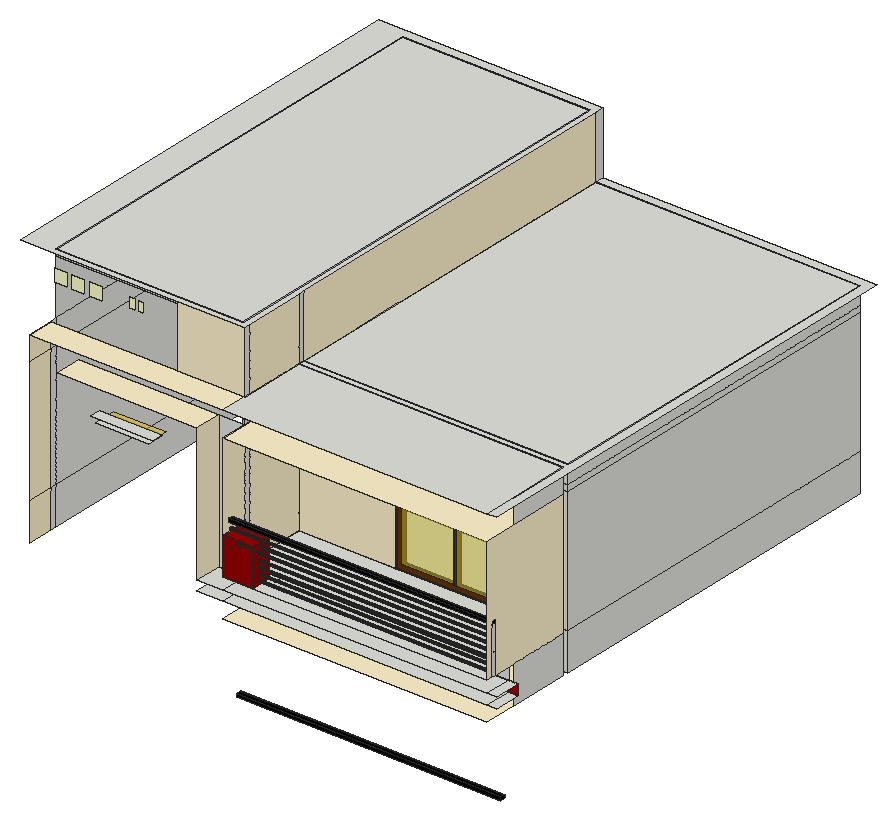
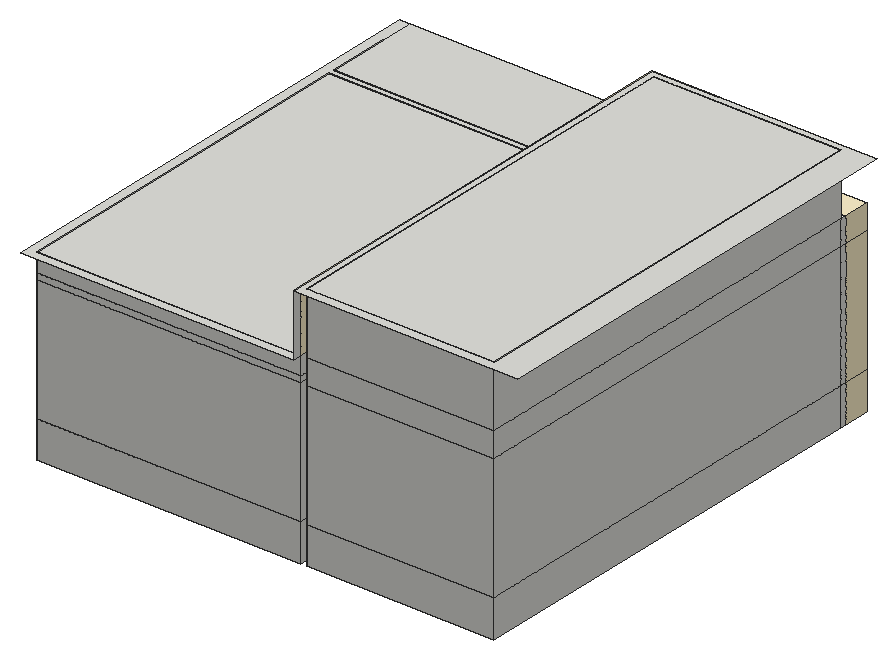
# SketchUp Ruby script. Lengths in inches.
U = 1.inch
M = Sketchup.active_model
def pt(a) = Geom::Point3d.new(a.map { |v| v * U })
def face(e, loops, mat)
  f = e.add_face(loops[0].map { |a| pt(a) })
  loops[1..].each { |l| e.add_face(l.map { |a| pt(a) }).erase! }
  f.material = f.back_material = mat if mat
  f
end
# faces: each face lists its corners as indices into pts; further lists are holes
def faces(e, pts, list, mat = nil) = list.each { |f| face(e, (f[0].is_a?(Array) ? f : [f]).map { |l| l.map { |i| pts[i] } }, mat) }
# xy, xz, yz: faces in a plane at the given z, y or x. An outline is a flat list of corners, or four numbers for a rectangle; further outlines are holes
def ring(l) = l.size == 4 ? [[l[0], l[1]], [l[2], l[1]], [l[2], l[3]], [l[0], l[3]]] : l.each_slice(2).to_a
def flat(e, list, mat, &to3) = list.each { |f| face(e, (f[0].is_a?(Array) ? f : [f]).map { |l| ring(l).map { |u, v| to3.(u, v) } }, mat) }
def xy(e, z, list, mat = nil) = flat(e, list, mat) { |x, y| [x, y, z] }
def xz(e, y, list, mat = nil) = flat(e, list, mat) { |x, z| [x, y, z] }
def yz(e, x, list, mat = nil) = flat(e, list, mat) { |y, z| [x, y, z] }
def lines(e, pts, list) = list.each { |a, b| e.add_line(pt(pts[a]), pt(pts[b])) }
# prism: a flat outline (further loops are holes) pulled along v
def prism(e, loops, v, mat = nil)
  f = face(e, loops, mat); d = Geom::Vector3d.new(v.map { |x| x * U })
  f.pushpull(f.normal.samedirection?(d) ? d.length : -d.length)
end
def box(e, o, s, mat = nil) = prism(e, [[o, [o[0] + s[0], o[1], o[2]], [o[0] + s[0], o[1] + s[1], o[2]], [o[0], o[1] + s[1], o[2]]]], [0, 0, s[2]], mat)
def at(x, y, z, deg = 0) = Geom::Transformation.translation(pt([x, y, z])) * Geom::Transformation.rotation(ORIGIN, Z_AXIS, deg.degrees)
def axes(o, x, y, z) = Geom::Transformation.new([*x, 0, *y, 0, *z, 0, *pt(o).to_a, 1])
def part(name) = M.definitions.add(name)
# library, detail: a bought-in or finely detailed component or shape, given as its bounding box
def library(name, o, s) = part(name).tap { |d| box(d.entities, o, s) }
def detail(e, o, s) = box(e.add_group.entities, o, s)
def put(e, d, t, mat = nil) = e.add_instance(d, t).tap { |i| i.material = mat if mat }
def group(e, t, mat = nil) = e.add_group.tap { |g| g.transformation = t; g.material = mat if mat }.entities
root = M.entities
M.materials.add("[Color A07]").color = [153, 0, 0]
M.materials.add("[Color C08]").color = [102, 51, 0]
M.materials.add("[Color D01]").color = [255, 242, 204]
M.materials.add("[Color E01]").color = [255, 255, 204]
M.materials.add("[Color M09]").color = [0, 0, 0]
M.materials.add("[Translucent Glass Blue]").color = [253, 204, 30]
M.materials["[Translucent Glass Blue]"].alpha = 0.5
M.materials.add("[Translucent Glass Gray]").color = [238, 223, 60]
M.materials["[Translucent Glass Gray]"].alpha = 0.5
xy(root,203.98,[[216.3125,98.41,471,103.375]],"[Color M09]")
xy(root,206.875,[[216.3125,98.41,471,103.375]],"[Color M09]")
xy(root,250.47,[[266.86,173.875,320.67,179.875]])
xy(root,254.4375,[[363.24,173.875,420.42,179.875]])
xy(root,278.875,[[216.3125,82.5625,471,173.875]],"[Color D01]")
xy(root,293.6875,[[191.1875,82.5625,216.3125,108.25],[216.3125,82.5625,471,108.25],[471,82.5625,480,108.25]])
xy(root,303.625,[[191.1875,82.5625,216.3125,108.25],[216.3125,82.5625,471,108.25],[471,82.5625,480,108.25]])
xy(root,314.875,[[216.3125,82.5625,245.1875,101.8125],[245.1875,82.5625,471,82.5625,471,108.25,216.3125,108.25,216.3125,101.8125,245.1875,101.8125],[216.3125,108.25,471,173.875],[309.76,173.875,426.51,175.03],[309.76,179.125,426.51,179.875],
  [216.3125,179.875,471,531.625]])
xy(root,314.875,[[309.76,175.03,426.51,179.125]],"[Color C08]")
xy(root,319.09,[[314.82,175.03,364.56,179.125],[364.56,175.03,368.13,179.125],[368.13,175.03,421.45,179.125]],"[Color C08]")
xy(root,350.875,[[216.3125,82.5625,245.1875,101.8125]],"[Color A07]")
xy(root,359.85,[[216.3125,88.6875,471,92.1875]],"[Color M09]")
xy(root,362.875,[[216.3125,88.6875,471,92.1875]],"[Color M09]")
xy(root,393.52,[[80.73,97.9375,131.98,114.25]])
xy(root,393.52,[[80.73,114.25,131.98,120.5625]],"[Translucent Glass Blue]")
xy(root,397.86,[[76.39,97.9375,136.32,108.25]])
xy(root,407.97,[[314.82,175.03,364.56,179.125],[364.56,175.03,368.13,179.125],[368.13,175.03,421.45,179.125]],"[Color C08]")
xy(root,412.1875,[[309.76,173.875,426.51,175.03],[309.76,179.125,426.51,179.875]])
xy(root,412.1875,[[309.76,175.03,426.51,179.125]],"[Color C08]")
xy(root,434.875,[[56.54,82.5625,191.1875,108.25],[216.3125,82.5625,471,173.875]],"[Color D01]")
xy(root,441,[[216.3125,179.875,471,531.625]])
xy(root,458.875,[[216.3125,82.5625,471,173.875],[471,82.5625,480,82.5625,480,540.625,216.3125,540.625,216.3125,531.625,471,531.625,471,179.875,216.3125,179.875,216.3125,173.875,471,173.875],[216.3125,179.875,471,531.625]])
xy(root,458.875,[[29.875,82.5625,216.3125,108.25]],"[Color D01]")
xy(root,512.875,[[29.875,114.25,210.3125,531.625]])
xy(root,518.875,[[0,108.25,29.875,108.25,29.875,531.625,210.3125,531.625,210.3125,114.25,29.875,114.25,29.875,108.25,216.3125,108.25,216.3125,540.625,0,540.625],[29.875,114.25,210.3125,531.625]])
xz(root,82.5625,[[216.3125,314.875,245.1875,350.875]],"[Color A07]")
xz(root,88.6875,[[216.3125,359.85,471,362.875]],"[Color M09]")
xz(root,92.1875,[[216.3125,359.85,471,362.875]],"[Color M09]")
xz(root,98.41,[[216.3125,203.98,471,206.875]],"[Color M09]")
xz(root,101.8125,[[216.3125,314.875,245.1875,350.875]],"[Color A07]")
xz(root,103.375,[[216.3125,203.98,471,206.875]],"[Color M09]")
xz(root,108.25,[[191.1875,303.625,216.3125,434.875],[216.3125,303.625,471,314.875]])
xz(root,108.25,[[191.1875,293.6875,480,303.625]],"[Color A07]")
xz(root,108.25,[[152.27,458.875,216.3125,518.875]],"[Color D01]")
xz(root,108.25,[[33.0625,493.93,45.1875,506.06],[49.25,493.93,61.375,506.06],[66.875,493.93,79,506.06],[105.77,497.1,110.39,506.41],[113.89,497.1,118.52,506.41]],"[Color E01]")
xz(root,114.25,[[29.875,512.875,210.3125,518.875]])
xz(root,173.875,[[216.3125,278.875,471,314.875],[216.3125,434.875,471,458.875]])
xz(root,173.875,[[216.3125,314.875,309.76,314.875,309.76,412.1875,426.51,412.1875,426.51,314.875,471,314.875,471,434.875,216.3125,434.875]],"[Color D01]")
xz(root,175.03,[[[309.76,314.875,426.51,412.1875],[314.82,319.09,421.45,407.97]],[364.56,319.09,368.13,407.97]],"[Color C08]")
xz(root,175.03,[[314.82,319.09,364.56,407.97],[368.13,319.09,421.45,407.97]],"[Translucent Glass Gray]")
xz(root,179.125,[[[309.76,314.875,426.51,412.1875],[314.82,319.09,421.45,407.97]],[364.56,319.09,368.13,407.97]],"[Color C08]")
xz(root,179.875,[[216.3125,278.875,471,314.875],[216.3125,314.875,216.3125,434.875,471,434.875,471,314.875,426.51,314.875,426.51,412.1875,309.76,412.1875,309.76,314.875],[216.3125,434.875,471,441],[216.3125,441,471,458.875]])
xz(root,531.625,[[29.875,278.875,210.3125,314.875],[216.3125,278.875,471,314.875],[29.875,314.875,210.3125,434.875],[216.3125,314.875,471,434.875],[29.875,434.875,210.3125,458.875],
  [216.3125,434.875,471,441],[216.3125,441,471,458.875],[29.875,458.875,210.3125,512.875],[29.875,512.875,52.375,518.875],[52.375,512.875,210.3125,518.875]])
yz(root,29.875,[[108.25,278.875,114.25,314.875],[114.25,278.875,531.625,314.875],[108.25,314.875,114.25,434.875],[114.25,314.875,531.625,434.875],[108.25,434.875,114.25,458.875],
  [114.25,434.875,531.625,458.875],[114.25,458.875,531.625,512.875],[114.25,512.875,531.625,518.875]])
yz(root,29.875,[[82.5625,278.875,108.25,314.875],[82.5625,314.875,108.25,434.875],[82.5625,434.875,108.25,458.875]],"[Color D01]")
yz(root,191.1875,[[82.5625,303.625,108.25,434.875]],"[Color D01]")
yz(root,210.3125,[[114.25,278.875,531.625,314.875],[114.25,314.875,531.625,434.875],[114.25,434.875,531.625,458.875],[114.25,458.875,531.625,512.875],[114.25,512.875,531.625,518.875]])
yz(root,216.3125,[[114.25,278.875,173.875,296.875],[173.875,278.875,179.875,296.875],[179.875,278.875,531.625,314.875],[114.25,296.875,173.875,314.875],[173.875,296.875,179.875,458.875],
  [[82.5625,314.875,101.8125,350.875],[90.49,334.97,90.26,335,90.05,335.09,89.87,335.23,89.73,335.41,89.64,335.62,89.61,335.85,89.64,336.07,89.73,336.28,89.87,336.47,90.05,336.6,90.26,336.69,90.49,336.72,90.71,336.69,90.93,336.6,91.11,336.47,91.25,336.28,91.33,336.07,91.36,335.85,91.33,335.62,91.25,335.41,91.11,335.23,90.93,335.09,90.71,335]],[108.25,314.875,114.25,434.875],[179.875,314.875,531.625,434.875],[108.25,434.875,114.25,458.875],[114.25,434.875,173.875,458.875],
  [179.875,434.875,531.625,441],[179.875,441,240.8,458.875],[240.8,441,293.43,458.875],[293.43,441,531.625,458.875],[108.25,458.875,114.25,518.875],
  [173.875,458.875,179.875,518.875],[531.625,458.875,540.625,518.875]])
yz(root,216.3125,[[[101.8125,314.875,108.25,314.875,108.25,434.875,82.5625,434.875,82.5625,350.875,101.8125,350.875],[88.6875,359.85,92.1875,362.875],[90.49,352.97,90.26,353,90.05,353.09,89.87,353.23,89.73,353.41,89.64,353.62,89.61,353.85,89.64,354.07,89.73,354.28,89.87,354.47,90.05,354.6,90.26,354.69,90.49,354.72,90.71,354.69,90.93,354.6,91.11,354.47,91.25,354.28,91.33,354.07,91.36,353.85,91.33,353.62,91.25,353.41,91.11,353.23,90.93,353.09,90.71,353]],[114.25,314.875,173.875,434.875],[114.25,458.875,173.875,518.875],[179.875,458.875,531.625,518.875]],"[Color D01]")
yz(root,222.125,[[90.49,340.97,90.26,341,90.05,341.09,89.87,341.23,89.73,341.41,89.64,341.62,89.61,341.85,89.64,342.07,89.73,342.28,89.87,342.47,90.05,342.6,90.26,342.69,90.49,342.72,90.71,342.69,90.93,342.6,91.11,342.47,91.25,342.28,91.33,342.07,91.36,341.85,91.33,341.62,91.25,341.41,91.11,341.23,90.93,341.09,90.71,341]],"[Color M09]")
yz(root,244,[[90.49,328.97,90.26,329,90.05,329.09,89.87,329.23,89.73,329.41,89.64,329.62,89.61,329.85,89.64,330.07,89.73,330.28,89.87,330.47,90.05,330.6,90.26,330.69,90.49,330.72,90.71,330.69,90.93,330.6,91.11,330.47,91.25,330.28,91.33,330.07,91.36,329.85,91.33,329.62,91.25,329.41,91.11,329.23,90.93,329.09,90.71,329]],"[Color M09]")
yz(root,244.8125,[[90.49,322.97,90.26,323,90.05,323.09,89.87,323.23,89.73,323.41,89.64,323.62,89.61,323.85,89.64,324.07,89.73,324.28,89.87,324.47,90.05,324.6,90.26,324.69,90.49,324.72,90.71,324.69,90.93,324.6,91.11,324.47,91.25,324.28,91.33,324.07,91.36,323.85,91.33,323.62,91.25,323.41,91.11,323.23,90.93,323.09,90.71,323]],"[Color M09]")
yz(root,245.1875,[[[82.5625,314.875,101.8125,350.875],[90.49,316.97,90.26,317,90.05,317.09,89.87,317.23,89.73,317.41,89.64,317.62,89.61,317.85,89.64,318.07,89.73,318.28,89.87,318.47,90.05,318.6,90.26,318.69,90.49,318.72,90.71,318.69,90.93,318.6,91.11,318.47,91.25,318.28,91.33,318.07,91.36,317.85,91.33,317.62,91.25,317.41,91.11,317.23,90.93,317.09,90.71,317],[90.49,346.97,90.26,347,90.05,347.09,89.87,347.23,89.73,347.41,89.64,347.62,89.61,347.85,89.64,348.07,89.73,348.28,89.87,348.47,90.05,348.6,90.26,348.69,90.49,348.72,90.71,348.69,90.93,348.6,91.11,348.47,91.25,348.28,91.33,348.07,91.36,347.85,91.33,347.62,91.25,347.41,91.11,347.23,90.93,347.09,90.71,347]]],"[Color A07]")
yz(root,261.375,[[90.49,322.97,90.71,323,90.93,323.09,91.11,323.23,91.25,323.41,91.33,323.62,91.36,323.85,91.33,324.07,91.25,324.28,91.11,324.47,90.93,324.6,90.71,324.69,90.49,324.72,90.26,324.69,90.05,324.6,89.87,324.47,89.73,324.28,89.64,324.07,89.61,323.85,89.64,323.62,89.73,323.41,89.87,323.23,90.05,323.09,90.26,323]],"[Color M09]")
yz(root,309.76,[[173.875,314.875,175.03,412.1875],[179.125,314.875,179.875,412.1875]])
yz(root,309.76,[[175.03,314.875,179.125,412.1875]],"[Color C08]")
yz(root,314.82,[[175.03,319.09,179.125,407.97]],"[Color C08]")
yz(root,364.56,[[175.03,319.09,179.125,407.97]],"[Color C08]")
yz(root,368.13,[[175.03,319.09,179.125,407.97]],"[Color C08]")
yz(root,421.45,[[175.03,319.09,179.125,407.97]],"[Color C08]")
yz(root,426.51,[[173.875,314.875,175.03,412.1875],[179.125,314.875,179.875,412.1875]])
yz(root,426.51,[[175.03,314.875,179.125,412.1875]],"[Color C08]")
yz(root,471,[[114.25,278.875,173.875,314.875],[179.875,278.875,531.625,314.875],[[88.6875,314.875,92.1875,359.85],[90.49,346.97,90.71,347,90.93,347.09,91.11,347.23,91.25,347.41,91.33,347.62,91.36,347.85,91.33,348.07,91.25,348.28,91.11,348.47,90.93,348.6,90.71,348.69,90.49,348.72,90.26,348.69,90.05,348.6,89.87,348.47,89.73,348.28,89.64,348.07,89.61,347.85,89.64,347.62,89.73,347.41,89.87,347.23,90.05,347.09,90.26,347],[90.49,340.97,90.71,341,90.93,341.09,91.11,341.23,91.25,341.41,91.33,341.62,91.36,341.85,91.33,342.07,91.25,342.28,91.11,342.47,90.93,342.6,90.71,342.69,90.49,342.72,90.26,342.69,90.05,342.6,89.87,342.47,89.73,342.28,89.64,342.07,89.61,341.85,89.64,341.62,89.73,341.41,89.87,341.23,90.05,341.09,90.26,341],[90.49,334.97,90.71,335,90.93,335.09,91.11,335.23,91.25,335.41,91.33,335.62,91.36,335.85,91.33,336.07,91.25,336.28,91.11,336.47,90.93,336.6,90.71,336.69,90.49,336.72,90.26,336.69,90.05,336.6,89.87,336.47,89.73,336.28,89.64,336.07,89.61,335.85,89.64,335.62,89.73,335.41,89.87,335.23,90.05,335.09,90.26,335],[90.49,328.97,90.71,329,90.93,329.09,91.11,329.23,91.25,329.41,91.33,329.62,91.36,329.85,91.33,330.07,91.25,330.28,91.11,330.47,90.93,330.6,90.71,330.69,90.49,330.72,90.26,330.69,90.05,330.6,89.87,330.47,89.73,330.28,89.64,330.07,89.61,329.85,89.64,329.62,89.73,329.41,89.87,329.23,90.05,329.09,90.26,329],[90.49,322.97,90.71,323,90.93,323.09,91.11,323.23,91.25,323.41,91.33,323.62,91.36,323.85,91.33,324.07,91.25,324.28,91.11,324.47,90.93,324.6,90.71,324.69,90.49,324.72,90.26,324.69,90.05,324.6,89.87,324.47,89.73,324.28,89.64,324.07,89.61,323.85,89.64,323.62,89.73,323.41,89.87,323.23,90.05,323.09,90.26,323],[90.49,316.97,90.71,317,90.93,317.09,91.11,317.23,91.25,317.41,91.33,317.62,91.36,317.85,91.33,318.07,91.25,318.28,91.11,318.47,90.93,318.6,90.71,318.69,90.49,318.72,90.26,318.69,90.05,318.6,89.87,318.47,89.73,318.28,89.64,318.07,89.61,317.85,89.64,317.62,89.73,317.41,89.87,317.23,90.05,317.09,90.26,317],[90.49,352.97,90.71,353,90.93,353.09,91.11,353.23,91.25,353.41,91.33,353.62,91.36,353.85,91.33,354.07,91.25,354.28,91.11,354.47,90.93,354.6,90.71,354.69,90.49,354.72,90.26,354.69,90.05,354.6,89.87,354.47,89.73,354.28,89.64,354.07,89.61,353.85,89.64,353.62,89.73,353.41,89.87,353.23,90.05,353.09,90.26,353]],[179.875,314.875,531.625,434.875],[114.25,434.875,173.875,458.875],
  [179.875,434.875,531.625,441],[179.875,441,531.625,458.875]])
yz(root,471,[[82.5625,314.875,82.5625,434.875,173.875,434.875,173.875,314.875,92.1875,314.875,92.1875,362.875,88.6875,362.875,88.6875,314.875]],"[Color D01]")
yz(root,471,[[98.41,203.98,103.375,206.875],[90.49,316.97,90.71,317,90.93,317.09,91.11,317.23,91.25,317.41,91.33,317.62,91.36,317.85,91.33,318.07,91.25,318.28,91.11,318.47,90.93,318.6,90.71,318.69,90.49,318.72,90.26,318.69,90.05,318.6,89.87,318.47,89.73,318.28,89.64,318.07,89.61,317.85,89.64,317.62,89.73,317.41,89.87,317.23,90.05,317.09,90.26,317],[90.49,322.97,90.71,323,90.93,323.09,91.11,323.23,91.25,323.41,91.33,323.62,91.36,323.85,91.33,324.07,91.25,324.28,91.11,324.47,90.93,324.6,90.71,324.69,90.49,324.72,90.26,324.69,90.05,324.6,89.87,324.47,89.73,324.28,89.64,324.07,89.61,323.85,89.64,323.62,89.73,323.41,89.87,323.23,90.05,323.09,90.26,323],[90.49,328.97,90.71,329,90.93,329.09,91.11,329.23,91.25,329.41,91.33,329.62,91.36,329.85,91.33,330.07,91.25,330.28,91.11,330.47,90.93,330.6,90.71,330.69,90.49,330.72,90.26,330.69,90.05,330.6,89.87,330.47,89.73,330.28,89.64,330.07,89.61,329.85,89.64,329.62,89.73,329.41,89.87,329.23,90.05,329.09,90.26,329],[90.49,334.97,90.71,335,90.93,335.09,91.11,335.23,91.25,335.41,91.33,335.62,91.36,335.85,91.33,336.07,91.25,336.28,91.11,336.47,90.93,336.6,90.71,336.69,90.49,336.72,90.26,336.69,90.05,336.6,89.87,336.47,89.73,336.28,89.64,336.07,89.61,335.85,89.64,335.62,89.73,335.41,89.87,335.23,90.05,335.09,90.26,335],
  [90.49,340.97,90.71,341,90.93,341.09,91.11,341.23,91.25,341.41,91.33,341.62,91.36,341.85,91.33,342.07,91.25,342.28,91.11,342.47,90.93,342.6,90.71,342.69,90.49,342.72,90.26,342.69,90.05,342.6,89.87,342.47,89.73,342.28,89.64,342.07,89.61,341.85,89.64,341.62,89.73,341.41,89.87,341.23,90.05,341.09,90.26,341],[90.49,346.97,90.71,347,90.93,347.09,91.11,347.23,91.25,347.41,91.33,347.62,91.36,347.85,91.33,348.07,91.25,348.28,91.11,348.47,90.93,348.6,90.71,348.69,90.49,348.72,90.26,348.69,90.05,348.6,89.87,348.47,89.73,348.28,89.64,348.07,89.61,347.85,89.64,347.62,89.73,347.41,89.87,347.23,90.05,347.09,90.26,347],[90.49,352.97,90.71,353,90.93,353.09,91.11,353.23,91.25,353.41,91.33,353.62,91.36,353.85,91.33,354.07,91.25,354.28,91.11,354.47,90.93,354.6,90.71,354.69,90.49,354.72,90.26,354.69,90.05,354.6,89.87,354.47,89.73,354.28,89.64,354.07,89.61,353.85,89.64,353.62,89.73,353.41,89.87,353.23,90.05,353.09,90.26,353],[88.6875,359.85,92.1875,362.875]],"[Color M09]")
p = [[471,90.26,317],[471,90.05,317.09],[245.1875,90.05,317.09],[245.1875,90.26,317],[471,90.49,316.97],[245.1875,90.49,316.97],
  [471,90.71,317],[245.1875,90.71,317],[471,90.93,317.09],[245.1875,90.93,317.09],[471,89.87,317.23],[245.1875,89.87,317.23],
  [471,91.11,317.23],[245.1875,91.11,317.23],[471,89.73,317.41],[245.1875,89.73,317.41],[471,91.25,317.41],[245.1875,91.25,317.41],
  [471,89.64,317.62],[245.1875,89.64,317.62],[471,91.33,317.62],[245.1875,91.33,317.62],[471,89.61,317.85],[245.1875,89.61,317.85],
  [471,91.36,317.85],[245.1875,91.36,317.85],[471,89.64,318.07],[245.1875,89.64,318.07],[471,91.33,318.07],[245.1875,91.33,318.07],
  [471,89.73,318.28],[245.1875,89.73,318.28],[471,91.25,318.28],[245.1875,91.25,318.28],[471,89.87,318.47],[245.1875,89.87,318.47],
  [471,91.11,318.47],[245.1875,91.11,318.47],[471,90.05,318.6],[245.1875,90.05,318.6],[471,90.93,318.6],[245.1875,90.93,318.6],
  [471,90.26,318.69],[245.1875,90.26,318.69],[471,90.71,318.69],[245.1875,90.71,318.69],[471,90.49,318.72],[245.1875,90.49,318.72],
  [261.375,90.26,323],[261.375,90.05,323.09],[244.8125,90.05,323.09],[244.8125,90.26,323],[471,90.26,323],[471,90.05,323.09],
  [261.375,90.49,322.97],[244.8125,90.49,322.97],[471,90.49,322.97],[261.375,90.71,323],[244.8125,90.71,323],[471,90.71,323],
  [261.375,90.93,323.09],[244.8125,90.93,323.09],[471,90.93,323.09],[261.375,89.87,323.23],[244.8125,89.87,323.23],[471,89.87,323.23],
  [261.375,91.11,323.23],[244.8125,91.11,323.23],[471,91.11,323.23],[261.375,89.73,323.41],[244.8125,89.73,323.41],[471,89.73,323.41],
  [261.375,91.25,323.41],[244.8125,91.25,323.41],[471,91.25,323.41],[261.375,89.64,323.62],[244.8125,89.64,323.62],[471,89.64,323.62],
  [261.375,91.33,323.62],[244.8125,91.33,323.62],[471,91.33,323.62],[261.375,89.61,323.85],[244.8125,89.61,323.85],[471,89.61,323.85],
  [261.375,91.36,323.85],[244.8125,91.36,323.85],[471,91.36,323.85],[261.375,89.64,324.07],[244.8125,89.64,324.07],[471,89.64,324.07],
  [261.375,91.33,324.07],[244.8125,91.33,324.07],[471,91.33,324.07],[261.375,89.73,324.28],[244.8125,89.73,324.28],[471,89.73,324.28],
  [261.375,91.25,324.28],[244.8125,91.25,324.28],[471,91.25,324.28],[261.375,89.87,324.47],[244.8125,89.87,324.47],[471,89.87,324.47],
  [261.375,91.11,324.47],[244.8125,91.11,324.47],[471,91.11,324.47],[261.375,90.05,324.6],[244.8125,90.05,324.6],[471,90.05,324.6],
  [261.375,90.93,324.6],[244.8125,90.93,324.6],[471,90.93,324.6],[261.375,90.26,324.69],[244.8125,90.26,324.69],[471,90.26,324.69],
  [261.375,90.71,324.69],[244.8125,90.71,324.69],[471,90.71,324.69],[261.375,90.49,324.72],[244.8125,90.49,324.72],[471,90.49,324.72],
  [471,90.26,329],[471,90.05,329.09],[244,90.05,329.09],[244,90.26,329],[471,90.49,328.97],[244,90.49,328.97],
  [471,90.71,329],[244,90.71,329],[471,90.93,329.09],[244,90.93,329.09],[471,89.87,329.23],[244,89.87,329.23],
  [471,91.11,329.23],[244,91.11,329.23],[471,89.73,329.41],[244,89.73,329.41],[471,91.25,329.41],[244,91.25,329.41],
  [471,89.64,329.62],[244,89.64,329.62],[471,91.33,329.62],[244,91.33,329.62],[471,89.61,329.85],[244,89.61,329.85],
  [471,91.36,329.85],[244,91.36,329.85],[471,89.64,330.07],[244,89.64,330.07],[471,91.33,330.07],[244,91.33,330.07],
  [471,89.73,330.28],[244,89.73,330.28],[471,91.25,330.28],[244,91.25,330.28],[471,89.87,330.47],[244,89.87,330.47],
  [471,91.11,330.47],[244,91.11,330.47],[471,90.05,330.6],[244,90.05,330.6],[471,90.93,330.6],[244,90.93,330.6],
  [471,90.26,330.69],[244,90.26,330.69],[471,90.71,330.69],[244,90.71,330.69],[471,90.49,330.72],[244,90.49,330.72],
  [471,90.26,335],[471,90.05,335.09],[216.3125,90.05,335.09],[216.3125,90.26,335],[471,90.49,334.97],[216.3125,90.49,334.97],
  [471,90.71,335],[216.3125,90.71,335],[471,90.93,335.09],[216.3125,90.93,335.09],[471,89.87,335.23],[216.3125,89.87,335.23],
  [471,91.11,335.23],[216.3125,91.11,335.23],[471,89.73,335.41],[216.3125,89.73,335.41],[471,91.25,335.41],[216.3125,91.25,335.41],
  [471,89.64,335.62],[216.3125,89.64,335.62],[471,91.33,335.62],[216.3125,91.33,335.62],[471,89.61,335.85],[216.3125,89.61,335.85],
  [471,91.36,335.85],[216.3125,91.36,335.85],[471,89.64,336.07],[216.3125,89.64,336.07],[471,91.33,336.07],[216.3125,91.33,336.07],
  [471,89.73,336.28],[216.3125,89.73,336.28],[471,91.25,336.28],[216.3125,91.25,336.28],[471,89.87,336.47],[216.3125,89.87,336.47],
  [471,91.11,336.47],[216.3125,91.11,336.47],[471,90.05,336.6],[216.3125,90.05,336.6],[471,90.93,336.6],[216.3125,90.93,336.6],
  [471,90.26,336.69],[216.3125,90.26,336.69],[471,90.71,336.69],[216.3125,90.71,336.69],[471,90.49,336.72],[216.3125,90.49,336.72],
  [471,90.26,341],[471,90.05,341.09],[222.125,90.05,341.09],[222.125,90.26,341],[471,90.49,340.97],[222.125,90.49,340.97],
  [471,90.71,341],[222.125,90.71,341],[471,90.93,341.09],[222.125,90.93,341.09],[471,89.87,341.23],[222.125,89.87,341.23],
  [471,91.11,341.23],[222.125,91.11,341.23],[471,89.73,341.41],[222.125,89.73,341.41],[471,91.25,341.41],[222.125,91.25,341.41],
  [471,89.64,341.62],[222.125,89.64,341.62],[471,91.33,341.62],[222.125,91.33,341.62],[471,89.61,341.85],[222.125,89.61,341.85],
  [471,91.36,341.85],[222.125,91.36,341.85],[471,89.64,342.07],[222.125,89.64,342.07],[471,91.33,342.07],[222.125,91.33,342.07],
  [471,89.73,342.28],[222.125,89.73,342.28],[471,91.25,342.28],[222.125,91.25,342.28],[471,89.87,342.47],[222.125,89.87,342.47],
  [471,91.11,342.47],[222.125,91.11,342.47],[471,90.05,342.6],[222.125,90.05,342.6],[471,90.93,342.6],[222.125,90.93,342.6],
  [471,90.26,342.69],[222.125,90.26,342.69],[471,90.71,342.69],[222.125,90.71,342.69],[471,90.49,342.72],[222.125,90.49,342.72],
  [471,90.26,347],[471,90.05,347.09],[245.1875,90.05,347.09],[245.1875,90.26,347],[471,90.49,346.97],[245.1875,90.49,346.97],
  [471,90.71,347],[245.1875,90.71,347],[471,90.93,347.09],[245.1875,90.93,347.09],[471,89.87,347.23],[245.1875,89.87,347.23],
  [471,91.11,347.23],[245.1875,91.11,347.23],[471,89.73,347.41],[245.1875,89.73,347.41],[471,91.25,347.41],[245.1875,91.25,347.41],
  [471,89.64,347.62],[245.1875,89.64,347.62],[471,91.33,347.62],[245.1875,91.33,347.62],[471,89.61,347.85],[245.1875,89.61,347.85],
  [471,91.36,347.85],[245.1875,91.36,347.85],[471,89.64,348.07],[245.1875,89.64,348.07],[471,91.33,348.07],[245.1875,91.33,348.07],
  [471,89.73,348.28],[245.1875,89.73,348.28],[471,91.25,348.28],[245.1875,91.25,348.28],[471,89.87,348.47],[245.1875,89.87,348.47],
  [471,91.11,348.47],[245.1875,91.11,348.47],[471,90.05,348.6],[245.1875,90.05,348.6],[471,90.93,348.6],[245.1875,90.93,348.6],
  [471,90.26,348.69],[245.1875,90.26,348.69],[471,90.71,348.69],[245.1875,90.71,348.69],[471,90.49,348.72],[245.1875,90.49,348.72],
  [471,90.26,353],[471,90.05,353.09],[216.3125,90.05,353.09],[216.3125,90.26,353],[471,90.49,352.97],[216.3125,90.49,352.97],
  [471,90.71,353],[216.3125,90.71,353],[471,90.93,353.09],[216.3125,90.93,353.09],[471,89.87,353.23],[216.3125,89.87,353.23],
  [471,91.11,353.23],[216.3125,91.11,353.23],[471,89.73,353.41],[216.3125,89.73,353.41],[471,91.25,353.41],[216.3125,91.25,353.41],
  [471,89.64,353.62],[216.3125,89.64,353.62],[471,91.33,353.62],[216.3125,91.33,353.62],[471,89.61,353.85],[216.3125,89.61,353.85],
  [471,91.36,353.85],[216.3125,91.36,353.85],[471,89.64,354.07],[216.3125,89.64,354.07],[471,91.33,354.07],[216.3125,91.33,354.07],
  [471,89.73,354.28],[216.3125,89.73,354.28],[471,91.25,354.28],[216.3125,91.25,354.28],[471,89.87,354.47],[216.3125,89.87,354.47],
  [471,91.11,354.47],[216.3125,91.11,354.47],[471,90.05,354.6],[216.3125,90.05,354.6],[471,90.93,354.6],[216.3125,90.93,354.6],
  [471,90.26,354.69],[216.3125,90.26,354.69],[471,90.71,354.69],[216.3125,90.71,354.69],[471,90.49,354.72],[216.3125,90.49,354.72],
  [191.1875,278.125,296.875],[216.3125,278.125,296.875]]
faces(root,p,[[0,1,2,3],[4,0,3,5],[6,4,5,7],[8,6,7,9],[1,10,11,2],[12,8,9,13],[10,14,15,11],[16,12,13,17],
  [14,18,19,15],[20,16,17,21],[18,22,23,19],[24,20,21,25],[22,26,27,23],[28,24,25,29],[26,30,31,27],[32,28,29,33],
  [30,34,35,31],[36,32,33,37],[34,38,39,35],[40,36,37,41],[38,42,43,39],[44,40,41,45],[42,46,47,43],[46,44,45,47],
  [48,49,50,51],[52,53,49,48],[54,48,51,55],[56,52,48,54],[57,54,55,58],[59,56,54,57],[60,57,58,61],[62,59,57,60],
  [49,63,64,50],[53,65,63,49],[66,60,61,67],[68,62,60,66],[63,69,70,64],[65,71,69,63],[72,66,67,73],[74,68,66,72],
  [69,75,76,70],[71,77,75,69],[78,72,73,79],[80,74,72,78],[75,81,82,76],[77,83,81,75],[84,78,79,85],[86,80,78,84],
  [81,87,88,82],[83,89,87,81],[90,84,85,91],[92,86,84,90],[87,93,94,88],[89,95,93,87],[96,90,91,97],[98,92,90,96],
  [93,99,100,94],[95,101,99,93],[102,96,97,103],[104,98,96,102],[99,105,106,100],[101,107,105,99],[108,102,103,109],[110,104,102,108],
  [105,111,112,106],[107,113,111,105],[114,108,109,115],[116,110,108,114],[111,117,118,112],[113,119,117,111],[117,114,115,118],[119,116,114,117],
  [120,121,122,123],[124,120,123,125],[126,124,125,127],[128,126,127,129],[121,130,131,122],[132,128,129,133],[130,134,135,131],[136,132,133,137],
  [134,138,139,135],[140,136,137,141],[138,142,143,139],[144,140,141,145],[142,146,147,143],[148,144,145,149],[146,150,151,147],[152,148,149,153],
  [150,154,155,151],[156,152,153,157],[154,158,159,155],[160,156,157,161],[158,162,163,159],[164,160,161,165],[162,166,167,163],[166,164,165,167],
  [168,169,170,171],[172,168,171,173],[174,172,173,175],[176,174,175,177],[169,178,179,170],[180,176,177,181],[178,182,183,179],[184,180,181,185],
  [182,186,187,183],[188,184,185,189],[186,190,191,187],[192,188,189,193],[190,194,195,191],[196,192,193,197],[194,198,199,195],[200,196,197,201],
  [198,202,203,199],[204,200,201,205],[202,206,207,203],[208,204,205,209],[206,210,211,207],[212,208,209,213],[210,214,215,211],[214,212,213,215],
  [216,217,218,219],[220,216,219,221],[222,220,221,223],[224,222,223,225],[217,226,227,218],[228,224,225,229],[226,230,231,227],[232,228,229,233],
  [230,234,235,231],[236,232,233,237],[234,238,239,235],[240,236,237,241],[238,242,243,239],[244,240,241,245],[242,246,247,243],[248,244,245,249],
  [246,250,251,247],[252,248,249,253],[250,254,255,251],[256,252,253,257],[254,258,259,255],[260,256,257,261],[258,262,263,259],[262,260,261,263],
  [264,265,266,267],[268,264,267,269],[270,268,269,271],[272,270,271,273],[265,274,275,266],[276,272,273,277],[274,278,279,275],[280,276,277,281],
  [278,282,283,279],[284,280,281,285],[282,286,287,283],[288,284,285,289],[286,290,291,287],[292,288,289,293],[290,294,295,291],[296,292,293,297],
  [294,298,299,295],[300,296,297,301],[298,302,303,299],[304,300,301,305],[302,306,307,303],[308,304,305,309],[306,310,311,307],[310,308,309,311],
  [312,313,314,315],[316,312,315,317],[318,316,317,319],[320,318,319,321],[313,322,323,314],[324,320,321,325],[322,326,327,323],[328,324,325,329],
  [326,330,331,327],[332,328,329,333],[330,334,335,331],[336,332,333,337],[334,338,339,335],[340,336,337,341],[338,342,343,339],[344,340,341,345],
  [342,346,347,343],[348,344,345,349],[346,350,351,347],[352,348,349,353],[350,354,355,351],[356,352,353,357],[354,358,359,355],[358,356,357,359]],"[Color M09]")
lines(root,p,[[360,361]])
